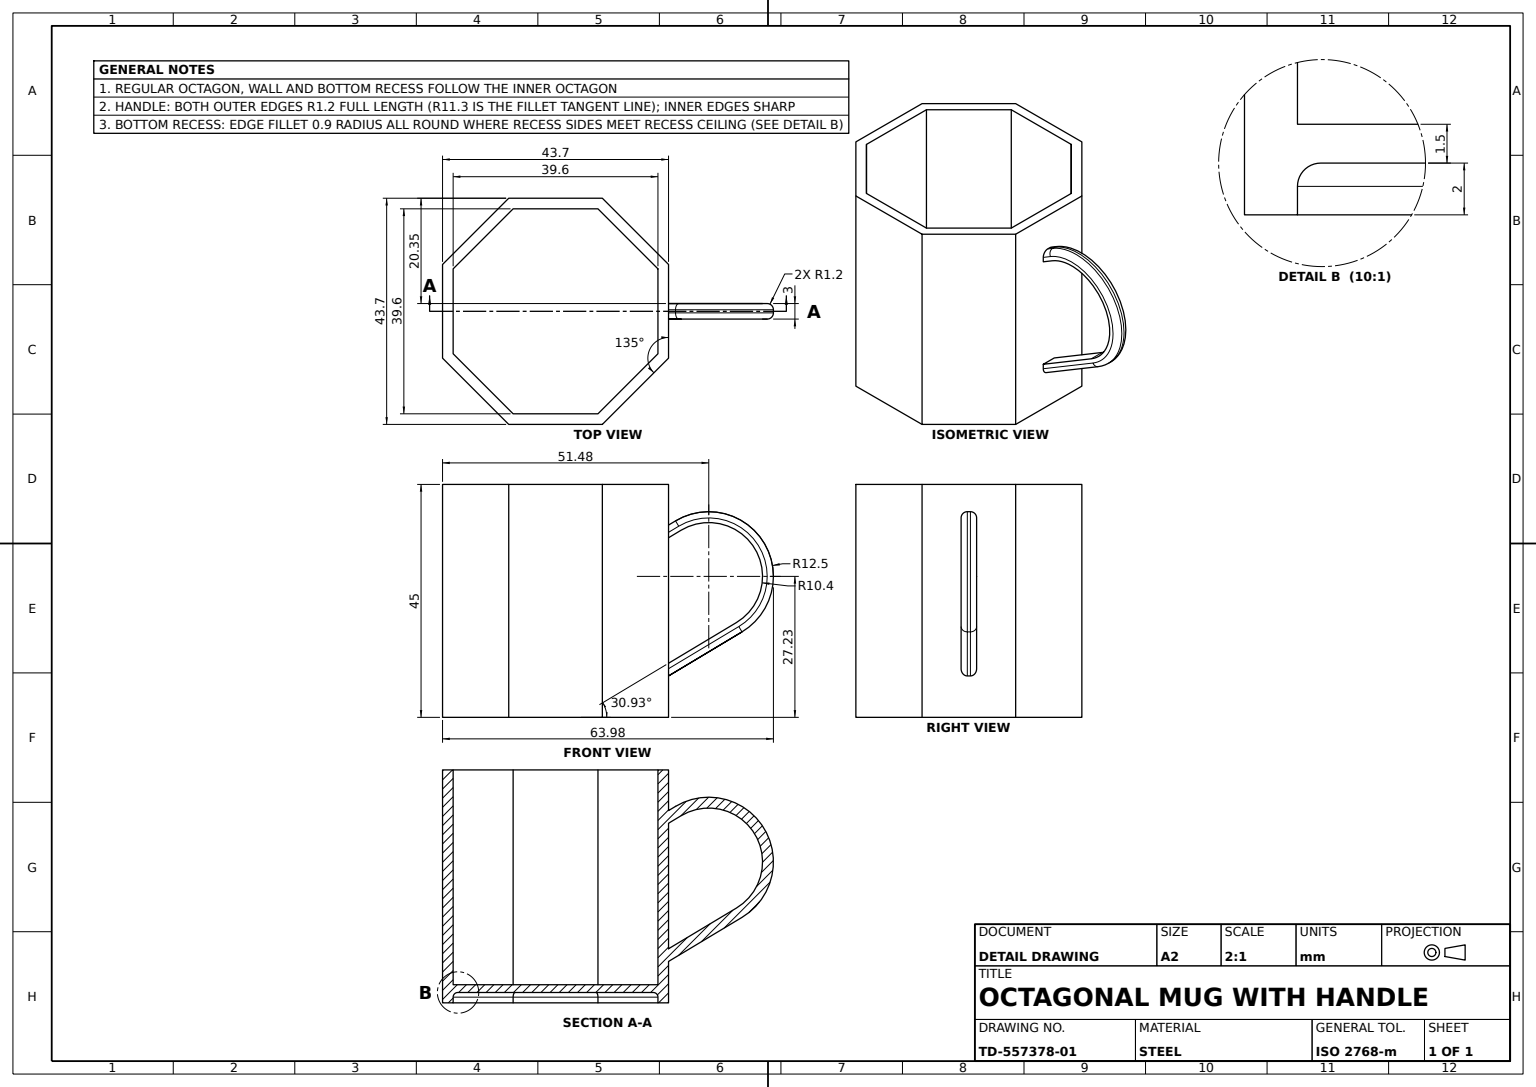
ISO-10303-21;
HEADER;
FILE_DESCRIPTION((''),'2;1');
FILE_NAME('','',(''),(''),'','','');
FILE_SCHEMA(('AUTOMOTIVE_DESIGN'));
ENDSEC;
DATA;
#1=APPLICATION_CONTEXT('');
#2=PRODUCT_CONTEXT('',#1,'mechanical');
#3=PRODUCT('','','',(#2));
#4=PRODUCT_DEFINITION_FORMATION('','',#3);
#5=PRODUCT_DEFINITION_CONTEXT('',#1,'design');
#6=PRODUCT_DEFINITION('','',#4,#5);
#7=PRODUCT_DEFINITION_SHAPE('','',#6);
#8=(LENGTH_UNIT()NAMED_UNIT(*)SI_UNIT(.MILLI.,.METRE.));
#9=(NAMED_UNIT(*)PLANE_ANGLE_UNIT()SI_UNIT($,.RADIAN.));
#10=(NAMED_UNIT(*)SI_UNIT($,.STERADIAN.)SOLID_ANGLE_UNIT());
#11=UNCERTAINTY_MEASURE_WITH_UNIT(LENGTH_MEASURE(1.E-05),#8,'distance_accuracy_value','');
#12=(GEOMETRIC_REPRESENTATION_CONTEXT(3)GLOBAL_UNCERTAINTY_ASSIGNED_CONTEXT((#11))GLOBAL_UNIT_ASSIGNED_CONTEXT((#8,#9,#10))REPRESENTATION_CONTEXT('',''));
#13=CARTESIAN_POINT('',(19.8,-21.4,8.201429));
#14=VERTEX_POINT('',#13);
#15=CARTESIAN_POINT('',(19.8,-22.5,8.201429));
#16=VERTEX_POINT('',#15);
#17=CARTESIAN_POINT('',(19.8,22.5,8.201429));
#18=DIRECTION('',(0.,-1.,0.));
#19=VECTOR('',#18,1000.);
#20=LINE('',#17,#19);
#21=EDGE_CURVE('',#14,#16,#20,.T.);
#22=ORIENTED_EDGE('',*,*,#21,.T.);
#23=CARTESIAN_POINT('',(8.201429,-22.5,19.8));
#24=VERTEX_POINT('',#23);
#25=DIRECTION('',(0.707106781,0.,-0.707106781));
#26=VECTOR('',#25,1000.);
#27=LINE('',#23,#26);
#28=EDGE_CURVE('',#24,#16,#27,.T.);
#29=ORIENTED_EDGE('',*,*,#28,.F.);
#30=CARTESIAN_POINT('',(8.201429,-21.4,19.8));
#31=VERTEX_POINT('',#30);
#32=CARTESIAN_POINT('',(8.201429,22.5,19.8));
#33=LINE('',#32,#19);
#34=EDGE_CURVE('',#31,#24,#33,.T.);
#35=ORIENTED_EDGE('',*,*,#34,.F.);
#36=LINE('',#30,#26);
#37=EDGE_CURVE('',#31,#14,#36,.T.);
#38=ORIENTED_EDGE('',*,*,#37,.T.);
#39=EDGE_LOOP('',(#22,#29,#35,#38));
#40=FACE_OUTER_BOUND('',#39,.T.);
#41=DIRECTION('',(-0.707106781,0.,-0.707106781));
#42=DIRECTION('',(-0.707106781,0.,0.707106781));
#43=AXIS2_PLACEMENT_3D('',#32,#41,#42);
#44=PLANE('',#43);
#45=ADVANCED_FACE('',(#40),#44,.T.);
#46=CARTESIAN_POINT('',(19.8,-21.4,-8.201429));
#47=VERTEX_POINT('',#46);
#48=CARTESIAN_POINT('',(8.201429,-21.4,-19.8));
#49=VERTEX_POINT('',#48);
#50=VECTOR('',#41,1000.);
#51=LINE('',#46,#50);
#52=EDGE_CURVE('',#47,#49,#51,.T.);
#53=ORIENTED_EDGE('',*,*,#52,.F.);
#54=CARTESIAN_POINT('',(18.9,-20.5,-7.828636));
#55=VERTEX_POINT('',#54);
#56=CARTESIAN_POINT('',(19.8,-20.872792,-8.201429));
#57=CARTESIAN_POINT('',(19.427208,-20.5,-8.047013));
#58=(BOUNDED_CURVE()B_SPLINE_CURVE(3,(#46,#56,#57,#54),.UNSPECIFIED.,.F.,.F.)B_SPLINE_CURVE_WITH_KNOTS((4,4),(0.,1.570796327),.UNSPECIFIED.)CURVE()GEOMETRIC_REPRESENTATION_ITEM()RATIONAL_B_SPLINE_CURVE((1.,0.804737854,0.804737854,1.))REPRESENTATION_ITEM(''));
#59=EDGE_CURVE('',#47,#55,#58,.T.);
#60=ORIENTED_EDGE('',*,*,#59,.T.);
#61=CARTESIAN_POINT('',(7.828636,-20.5,-18.9));
#62=VERTEX_POINT('',#61);
#63=CARTESIAN_POINT('',(13.364318,-20.5,-13.364318));
#64=DIRECTION('',(0.707106781,0.,0.707106781));
#65=VECTOR('',#64,1000.);
#66=LINE('',#63,#65);
#67=EDGE_CURVE('',#62,#55,#66,.T.);
#68=ORIENTED_EDGE('',*,*,#67,.F.);
#69=CARTESIAN_POINT('',(8.201429,-20.872792,-19.8));
#70=CARTESIAN_POINT('',(8.047013,-20.5,-19.427208));
#71=(BOUNDED_CURVE()B_SPLINE_CURVE(3,(#48,#69,#70,#61),.UNSPECIFIED.,.F.,.F.)B_SPLINE_CURVE_WITH_KNOTS((4,4),(0.,1.570796327),.UNSPECIFIED.)CURVE()GEOMETRIC_REPRESENTATION_ITEM()RATIONAL_B_SPLINE_CURVE((1.,0.804737854,0.804737854,1.))REPRESENTATION_ITEM(''));
#72=EDGE_CURVE('',#49,#62,#71,.T.);
#73=ORIENTED_EDGE('',*,*,#72,.F.);
#74=EDGE_LOOP('',(#53,#60,#68,#73));
#75=FACE_OUTER_BOUND('',#74,.T.);
#76=CARTESIAN_POINT('',(19.163604,-21.4,-7.565032));
#77=AXIS2_PLACEMENT_3D('',#76,#41,#42);
#78=CYLINDRICAL_SURFACE('',#77,0.9);
#79=ADVANCED_FACE('',(#75),#78,.F.);
#80=CARTESIAN_POINT('',(-8.201429,22.5,19.8));
#81=VERTEX_POINT('',#80);
#82=VERTEX_POINT('',#32);
#83=DIRECTION('',(1.,0.,0.));
#84=VECTOR('',#83,1000.);
#85=LINE('',#80,#84);
#86=EDGE_CURVE('',#81,#82,#85,.T.);
#87=ORIENTED_EDGE('',*,*,#86,.F.);
#88=CARTESIAN_POINT('',(-19.8,22.5,8.201429));
#89=VERTEX_POINT('',#88);
#90=LINE('',#88,#65);
#91=EDGE_CURVE('',#89,#81,#90,.T.);
#92=ORIENTED_EDGE('',*,*,#91,.F.);
#93=CARTESIAN_POINT('',(-19.8,22.5,-8.201429));
#94=VERTEX_POINT('',#93);
#95=DIRECTION('',(0.,0.,1.));
#96=VECTOR('',#95,1000.);
#97=LINE('',#93,#96);
#98=EDGE_CURVE('',#94,#89,#97,.T.);
#99=ORIENTED_EDGE('',*,*,#98,.F.);
#100=CARTESIAN_POINT('',(-8.201429,22.5,-19.8));
#101=VERTEX_POINT('',#100);
#102=VECTOR('',#42,1000.);
#103=LINE('',#100,#102);
#104=EDGE_CURVE('',#101,#94,#103,.T.);
#105=ORIENTED_EDGE('',*,*,#104,.F.);
#106=CARTESIAN_POINT('',(8.201429,22.5,-19.8));
#107=VERTEX_POINT('',#106);
#108=DIRECTION('',(-1.,0.,0.));
#109=VECTOR('',#108,1000.);
#110=LINE('',#106,#109);
#111=EDGE_CURVE('',#107,#101,#110,.T.);
#112=ORIENTED_EDGE('',*,*,#111,.F.);
#113=CARTESIAN_POINT('',(19.8,22.5,-8.201429));
#114=VERTEX_POINT('',#113);
#115=LINE('',#113,#50);
#116=EDGE_CURVE('',#114,#107,#115,.T.);
#117=ORIENTED_EDGE('',*,*,#116,.F.);
#118=VERTEX_POINT('',#17);
#119=DIRECTION('',(0.,0.,-1.));
#120=VECTOR('',#119,1000.);
#121=LINE('',#17,#120);
#122=EDGE_CURVE('',#118,#114,#121,.T.);
#123=ORIENTED_EDGE('',*,*,#122,.F.);
#124=LINE('',#32,#26);
#125=EDGE_CURVE('',#82,#118,#124,.T.);
#126=ORIENTED_EDGE('',*,*,#125,.F.);
#127=EDGE_LOOP('',(#87,#92,#99,#105,#112,#117,#123,#126));
#128=FACE_BOUND('',#127,.T.);
#129=CARTESIAN_POINT('',(9.05,22.5,21.848633));
#130=VERTEX_POINT('',#129);
#131=CARTESIAN_POINT('',(21.848633,22.5,9.05));
#132=VERTEX_POINT('',#131);
#133=LINE('',#129,#26);
#134=EDGE_CURVE('',#130,#132,#133,.T.);
#135=ORIENTED_EDGE('',*,*,#134,.T.);
#136=CARTESIAN_POINT('',(21.848633,22.5,-9.05));
#137=VERTEX_POINT('',#136);
#138=LINE('',#131,#120);
#139=EDGE_CURVE('',#132,#137,#138,.T.);
#140=ORIENTED_EDGE('',*,*,#139,.T.);
#141=CARTESIAN_POINT('',(9.05,22.5,-21.848633));
#142=VERTEX_POINT('',#141);
#143=LINE('',#136,#50);
#144=EDGE_CURVE('',#137,#142,#143,.T.);
#145=ORIENTED_EDGE('',*,*,#144,.T.);
#146=CARTESIAN_POINT('',(-9.05,22.5,-21.848633));
#147=VERTEX_POINT('',#146);
#148=LINE('',#141,#109);
#149=EDGE_CURVE('',#142,#147,#148,.T.);
#150=ORIENTED_EDGE('',*,*,#149,.T.);
#151=CARTESIAN_POINT('',(-21.848633,22.5,-9.05));
#152=VERTEX_POINT('',#151);
#153=LINE('',#146,#102);
#154=EDGE_CURVE('',#147,#152,#153,.T.);
#155=ORIENTED_EDGE('',*,*,#154,.T.);
#156=CARTESIAN_POINT('',(-21.848633,22.5,9.05));
#157=VERTEX_POINT('',#156);
#158=LINE('',#151,#96);
#159=EDGE_CURVE('',#152,#157,#158,.T.);
#160=ORIENTED_EDGE('',*,*,#159,.T.);
#161=CARTESIAN_POINT('',(-9.05,22.5,21.848633));
#162=VERTEX_POINT('',#161);
#163=LINE('',#156,#65);
#164=EDGE_CURVE('',#157,#162,#163,.T.);
#165=ORIENTED_EDGE('',*,*,#164,.T.);
#166=LINE('',#161,#84);
#167=EDGE_CURVE('',#162,#130,#166,.T.);
#168=ORIENTED_EDGE('',*,*,#167,.T.);
#169=EDGE_LOOP('',(#135,#140,#145,#150,#155,#160,#165,#168));
#170=FACE_OUTER_BOUND('',#169,.T.);
#171=CARTESIAN_POINT('',(0.,22.5,0.));
#172=DIRECTION('',(0.,1.,0.));
#173=AXIS2_PLACEMENT_3D('',#171,#172,#95);
#174=PLANE('',#173);
#175=ADVANCED_FACE('',(#128,#170),#174,.T.);
#176=CARTESIAN_POINT('',(-21.848633,-22.5,9.05));
#177=VERTEX_POINT('',#176);
#178=CARTESIAN_POINT('',(-9.05,-22.5,21.848633));
#179=VERTEX_POINT('',#178);
#180=LINE('',#176,#65);
#181=EDGE_CURVE('',#177,#179,#180,.T.);
#182=ORIENTED_EDGE('',*,*,#181,.T.);
#183=LINE('',#161,#19);
#184=EDGE_CURVE('',#162,#179,#183,.T.);
#185=ORIENTED_EDGE('',*,*,#184,.F.);
#186=ORIENTED_EDGE('',*,*,#164,.F.);
#187=LINE('',#156,#19);
#188=EDGE_CURVE('',#157,#177,#187,.T.);
#189=ORIENTED_EDGE('',*,*,#188,.T.);
#190=EDGE_LOOP('',(#182,#185,#186,#189));
#191=FACE_OUTER_BOUND('',#190,.T.);
#192=AXIS2_PLACEMENT_3D('',#156,#25,#41);
#193=PLANE('',#192);
#194=ADVANCED_FACE('',(#191),#193,.F.);
#195=CARTESIAN_POINT('',(36.05233,-5.989286,0.3));
#196=VERTEX_POINT('',#195);
#197=CARTESIAN_POINT('',(36.05233,-5.989286,-0.3));
#198=VERTEX_POINT('',#197);
#199=CARTESIAN_POINT('',(36.05233,-5.989286,1.5));
#200=LINE('',#199,#120);
#201=EDGE_CURVE('',#196,#198,#200,.T.);
#202=ORIENTED_EDGE('',*,*,#201,.F.);
#203=CARTESIAN_POINT('',(21.848633,-14.5,0.3));
#204=VERTEX_POINT('',#203);
#205=DIRECTION('',(-0.857799295,-0.513984796,0.));
#206=VECTOR('',#205,1000.);
#207=LINE('',#203,#206);
#208=EDGE_CURVE('',#196,#204,#207,.T.);
#209=ORIENTED_EDGE('',*,*,#208,.T.);
#210=CARTESIAN_POINT('',(21.848633,-14.5,-0.3));
#211=VERTEX_POINT('',#210);
#212=CARTESIAN_POINT('',(21.848633,-14.5,1.5));
#213=LINE('',#212,#120);
#214=EDGE_CURVE('',#204,#211,#213,.T.);
#215=ORIENTED_EDGE('',*,*,#214,.T.);
#216=DIRECTION('',(0.857799295,0.513984796,0.));
#217=VECTOR('',#216,1000.);
#218=LINE('',#210,#217);
#219=EDGE_CURVE('',#211,#198,#218,.T.);
#220=ORIENTED_EDGE('',*,*,#219,.T.);
#221=EDGE_LOOP('',(#202,#209,#215,#220));
#222=FACE_OUTER_BOUND('',#221,.T.);
#223=DIRECTION('',(-0.513984796,0.857799295,0.));
#224=AXIS2_PLACEMENT_3D('',#212,#223,#205);
#225=PLANE('',#224);
#226=ADVANCED_FACE('',(#222),#225,.F.);
#227=CARTESIAN_POINT('',(8.201429,-22.5,-19.8));
#228=VERTEX_POINT('',#227);
#229=LINE('',#106,#19);
#230=EDGE_CURVE('',#49,#228,#229,.T.);
#231=ORIENTED_EDGE('',*,*,#230,.F.);
#232=CARTESIAN_POINT('',(-8.201429,-21.4,-19.8));
#233=VERTEX_POINT('',#232);
#234=LINE('',#48,#109);
#235=EDGE_CURVE('',#49,#233,#234,.T.);
#236=ORIENTED_EDGE('',*,*,#235,.T.);
#237=CARTESIAN_POINT('',(-8.201429,-22.5,-19.8));
#238=VERTEX_POINT('',#237);
#239=LINE('',#100,#19);
#240=EDGE_CURVE('',#233,#238,#239,.T.);
#241=ORIENTED_EDGE('',*,*,#240,.T.);
#242=LINE('',#227,#109);
#243=EDGE_CURVE('',#228,#238,#242,.T.);
#244=ORIENTED_EDGE('',*,*,#243,.F.);
#245=EDGE_LOOP('',(#231,#236,#241,#244));
#246=FACE_OUTER_BOUND('',#245,.T.);
#247=AXIS2_PLACEMENT_3D('',#106,#95,#83);
#248=PLANE('',#247);
#249=ADVANCED_FACE('',(#246),#248,.T.);
#250=CARTESIAN_POINT('',(-19.8,-21.4,-8.201429));
#251=VERTEX_POINT('',#250);
#252=CARTESIAN_POINT('',(-19.8,-21.4,8.201429));
#253=VERTEX_POINT('',#252);
#254=LINE('',#250,#96);
#255=EDGE_CURVE('',#251,#253,#254,.T.);
#256=ORIENTED_EDGE('',*,*,#255,.T.);
#257=CARTESIAN_POINT('',(-19.8,-22.5,8.201429));
#258=VERTEX_POINT('',#257);
#259=LINE('',#88,#19);
#260=EDGE_CURVE('',#253,#258,#259,.T.);
#261=ORIENTED_EDGE('',*,*,#260,.T.);
#262=CARTESIAN_POINT('',(-19.8,-22.5,-8.201429));
#263=VERTEX_POINT('',#262);
#264=LINE('',#262,#96);
#265=EDGE_CURVE('',#263,#258,#264,.T.);
#266=ORIENTED_EDGE('',*,*,#265,.F.);
#267=LINE('',#93,#19);
#268=EDGE_CURVE('',#251,#263,#267,.T.);
#269=ORIENTED_EDGE('',*,*,#268,.F.);
#270=EDGE_LOOP('',(#256,#261,#266,#269));
#271=FACE_OUTER_BOUND('',#270,.T.);
#272=AXIS2_PLACEMENT_3D('',#93,#83,#119);
#273=PLANE('',#272);
#274=ADVANCED_FACE('',(#271),#273,.T.);
#275=CARTESIAN_POINT('',(-19.8,-19.,-8.201429));
#276=VERTEX_POINT('',#275);
#277=EDGE_CURVE('',#94,#276,#267,.T.);
#278=ORIENTED_EDGE('',*,*,#277,.T.);
#279=CARTESIAN_POINT('',(-8.201429,-19.,-19.8));
#280=VERTEX_POINT('',#279);
#281=LINE('',#279,#102);
#282=EDGE_CURVE('',#280,#276,#281,.T.);
#283=ORIENTED_EDGE('',*,*,#282,.F.);
#284=EDGE_CURVE('',#101,#280,#239,.T.);
#285=ORIENTED_EDGE('',*,*,#284,.F.);
#286=ORIENTED_EDGE('',*,*,#104,.T.);
#287=EDGE_LOOP('',(#278,#283,#285,#286));
#288=FACE_OUTER_BOUND('',#287,.T.);
#289=AXIS2_PLACEMENT_3D('',#100,#64,#25);
#290=PLANE('',#289);
#291=ADVANCED_FACE('',(#288),#290,.T.);
#292=CARTESIAN_POINT('',(-18.9,-20.5,-7.828636));
#293=VERTEX_POINT('',#292);
#294=CARTESIAN_POINT('',(-7.828636,-20.5,-18.9));
#295=VERTEX_POINT('',#294);
#296=CARTESIAN_POINT('',(-13.364318,-20.5,-13.364318));
#297=LINE('',#296,#26);
#298=EDGE_CURVE('',#293,#295,#297,.T.);
#299=ORIENTED_EDGE('',*,*,#298,.F.);
#300=CARTESIAN_POINT('',(-19.8,-20.872792,-8.201429));
#301=CARTESIAN_POINT('',(-19.427208,-20.5,-8.047013));
#302=(BOUNDED_CURVE()B_SPLINE_CURVE(3,(#250,#300,#301,#292),.UNSPECIFIED.,.F.,.F.)B_SPLINE_CURVE_WITH_KNOTS((4,4),(3.141592654,4.71238898),.UNSPECIFIED.)CURVE()GEOMETRIC_REPRESENTATION_ITEM()RATIONAL_B_SPLINE_CURVE((1.,0.804737854,0.804737854,1.))REPRESENTATION_ITEM(''));
#303=EDGE_CURVE('',#251,#293,#302,.T.);
#304=ORIENTED_EDGE('',*,*,#303,.F.);
#305=LINE('',#232,#102);
#306=EDGE_CURVE('',#233,#251,#305,.T.);
#307=ORIENTED_EDGE('',*,*,#306,.F.);
#308=CARTESIAN_POINT('',(-8.201429,-20.872792,-19.8));
#309=CARTESIAN_POINT('',(-8.047013,-20.5,-19.427208));
#310=(BOUNDED_CURVE()B_SPLINE_CURVE(3,(#232,#308,#309,#294),.UNSPECIFIED.,.F.,.F.)B_SPLINE_CURVE_WITH_KNOTS((4,4),(0.,1.570796327),.UNSPECIFIED.)CURVE()GEOMETRIC_REPRESENTATION_ITEM()RATIONAL_B_SPLINE_CURVE((1.,0.804737854,0.804737854,1.))REPRESENTATION_ITEM(''));
#311=EDGE_CURVE('',#233,#295,#310,.T.);
#312=ORIENTED_EDGE('',*,*,#311,.T.);
#313=EDGE_LOOP('',(#299,#304,#307,#312));
#314=FACE_OUTER_BOUND('',#313,.T.);
#315=CARTESIAN_POINT('',(-7.565032,-21.4,-19.163604));
#316=AXIS2_PLACEMENT_3D('',#315,#42,#64);
#317=CYLINDRICAL_SURFACE('',#316,0.9);
#318=ADVANCED_FACE('',(#314),#317,.F.);
#319=CARTESIAN_POINT('',(42.12752,4.733205,-0.3));
#320=VERTEX_POINT('',#319);
#321=CARTESIAN_POINT('',(29.62752,4.733205,-0.3));
#322=AXIS2_PLACEMENT_3D('',#321,#95,#83);
#323=CIRCLE('',#322,12.5);
#324=EDGE_CURVE('',#198,#320,#323,.T.);
#325=ORIENTED_EDGE('',*,*,#324,.F.);
#326=CARTESIAN_POINT('',(35.435548,-4.959927,-1.5));
#327=VERTEX_POINT('',#326);
#328=CARTESIAN_POINT('',(35.435548,-4.959927,-0.3));
#329=DIRECTION('',(0.513984796,-0.857799295,0.));
#330=AXIS2_PLACEMENT_3D('',#328,#205,#329);
#331=CIRCLE('',#330,1.2);
#332=EDGE_CURVE('',#327,#198,#331,.T.);
#333=ORIENTED_EDGE('',*,*,#332,.F.);
#334=CARTESIAN_POINT('',(40.92752,4.733205,-1.5));
#335=VERTEX_POINT('',#334);
#336=CARTESIAN_POINT('',(29.62752,4.733205,-1.5));
#337=AXIS2_PLACEMENT_3D('',#336,#119,#83);
#338=CIRCLE('',#337,11.3);
#339=EDGE_CURVE('',#335,#327,#338,.T.);
#340=ORIENTED_EDGE('',*,*,#339,.F.);
#341=CARTESIAN_POINT('',(40.92752,4.733205,-0.3));
#342=AXIS2_PLACEMENT_3D('',#341,#18,#119);
#343=CIRCLE('',#342,1.2);
#344=EDGE_CURVE('',#335,#320,#343,.T.);
#345=ORIENTED_EDGE('',*,*,#344,.T.);
#346=EDGE_LOOP('',(#325,#333,#340,#345));
#347=FACE_OUTER_BOUND('',#346,.T.);
#348=TOROIDAL_SURFACE('',#322,11.3,1.2);
#349=ADVANCED_FACE('',(#347),#348,.T.);
#350=ORIENTED_EDGE('',*,*,#260,.F.);
#351=CARTESIAN_POINT('',(-8.201429,-21.4,19.8));
#352=VERTEX_POINT('',#351);
#353=LINE('',#252,#65);
#354=EDGE_CURVE('',#253,#352,#353,.T.);
#355=ORIENTED_EDGE('',*,*,#354,.T.);
#356=CARTESIAN_POINT('',(-8.201429,-22.5,19.8));
#357=VERTEX_POINT('',#356);
#358=LINE('',#80,#19);
#359=EDGE_CURVE('',#352,#357,#358,.T.);
#360=ORIENTED_EDGE('',*,*,#359,.T.);
#361=LINE('',#257,#65);
#362=EDGE_CURVE('',#258,#357,#361,.T.);
#363=ORIENTED_EDGE('',*,*,#362,.F.);
#364=EDGE_LOOP('',(#350,#355,#360,#363));
#365=FACE_OUTER_BOUND('',#364,.T.);
#366=AXIS2_PLACEMENT_3D('',#88,#25,#41);
#367=PLANE('',#366);
#368=ADVANCED_FACE('',(#365),#367,.T.);
#369=CARTESIAN_POINT('',(21.848633,13.245418,1.5));
#370=VERTEX_POINT('',#369);
#371=CARTESIAN_POINT('',(21.848633,14.644347,0.3));
#372=VERTEX_POINT('',#371);
#373=CARTESIAN_POINT('',(21.848633,14.064891,1.5));
#374=CARTESIAN_POINT('',(21.848633,14.644347,1.002944));
#375=(BOUNDED_CURVE()B_SPLINE_CURVE(3,(#369,#373,#374,#371),.UNSPECIFIED.,.F.,.F.)B_SPLINE_CURVE_WITH_KNOTS((4,4),(4.71238898,6.283185307),.UNSPECIFIED.)CURVE()GEOMETRIC_REPRESENTATION_ITEM()RATIONAL_B_SPLINE_CURVE((1.,0.804737854,0.804737854,1.))REPRESENTATION_ITEM(''));
#376=EDGE_CURVE('',#370,#372,#375,.T.);
#377=ORIENTED_EDGE('',*,*,#376,.T.);
#378=CARTESIAN_POINT('',(21.848633,14.644347,-0.3));
#379=VERTEX_POINT('',#378);
#380=CARTESIAN_POINT('',(21.848633,14.644347,1.5));
#381=LINE('',#380,#120);
#382=EDGE_CURVE('',#372,#379,#381,.T.);
#383=ORIENTED_EDGE('',*,*,#382,.T.);
#384=CARTESIAN_POINT('',(21.848633,13.245418,-1.5));
#385=VERTEX_POINT('',#384);
#386=CARTESIAN_POINT('',(21.848633,14.644347,-1.002944));
#387=CARTESIAN_POINT('',(21.848633,14.064891,-1.5));
#388=(BOUNDED_CURVE()B_SPLINE_CURVE(3,(#378,#386,#387,#384),.UNSPECIFIED.,.F.,.T.)B_SPLINE_CURVE_WITH_KNOTS((4,4),(3.141592654,4.71238898),.UNSPECIFIED.)CURVE()GEOMETRIC_REPRESENTATION_ITEM()RATIONAL_B_SPLINE_CURVE((1.,0.804737854,0.804737854,1.))REPRESENTATION_ITEM(''));
#389=EDGE_CURVE('',#379,#385,#388,.T.);
#390=ORIENTED_EDGE('',*,*,#389,.T.);
#391=CARTESIAN_POINT('',(21.848633,12.196222,-1.5));
#392=VERTEX_POINT('',#391);
#393=LINE('',#391,#19);
#394=EDGE_CURVE('',#385,#392,#393,.T.);
#395=ORIENTED_EDGE('',*,*,#394,.T.);
#396=CARTESIAN_POINT('',(21.848633,12.196222,1.5));
#397=VERTEX_POINT('',#396);
#398=LINE('',#396,#120);
#399=EDGE_CURVE('',#397,#392,#398,.T.);
#400=ORIENTED_EDGE('',*,*,#399,.F.);
#401=LINE('',#396,#19);
#402=EDGE_CURVE('',#370,#397,#401,.T.);
#403=ORIENTED_EDGE('',*,*,#402,.F.);
#404=EDGE_LOOP('',(#377,#383,#390,#395,#400,#403));
#405=FACE_BOUND('',#404,.T.);
#406=CARTESIAN_POINT('',(21.848633,-22.5,9.05));
#407=VERTEX_POINT('',#406);
#408=CARTESIAN_POINT('',(21.848633,-22.5,-9.05));
#409=VERTEX_POINT('',#408);
#410=LINE('',#406,#120);
#411=EDGE_CURVE('',#407,#409,#410,.T.);
#412=ORIENTED_EDGE('',*,*,#411,.T.);
#413=LINE('',#136,#19);
#414=EDGE_CURVE('',#137,#409,#413,.T.);
#415=ORIENTED_EDGE('',*,*,#414,.F.);
#416=ORIENTED_EDGE('',*,*,#139,.F.);
#417=LINE('',#131,#19);
#418=EDGE_CURVE('',#132,#407,#417,.T.);
#419=ORIENTED_EDGE('',*,*,#418,.T.);
#420=EDGE_LOOP('',(#412,#415,#416,#419));
#421=FACE_OUTER_BOUND('',#420,.T.);
#422=CARTESIAN_POINT('',(21.848633,-13.101071,-1.5));
#423=VERTEX_POINT('',#422);
#424=CARTESIAN_POINT('',(21.848633,-13.920545,-1.5));
#425=CARTESIAN_POINT('',(21.848633,-14.5,-1.002944));
#426=(BOUNDED_CURVE()B_SPLINE_CURVE(3,(#422,#424,#425,#210),.UNSPECIFIED.,.F.,.F.)B_SPLINE_CURVE_WITH_KNOTS((4,4),(1.570796327,3.141592654),.UNSPECIFIED.)CURVE()GEOMETRIC_REPRESENTATION_ITEM()RATIONAL_B_SPLINE_CURVE((1.,0.804737854,0.804737854,1.))REPRESENTATION_ITEM(''));
#427=EDGE_CURVE('',#423,#211,#426,.T.);
#428=ORIENTED_EDGE('',*,*,#427,.T.);
#429=ORIENTED_EDGE('',*,*,#214,.F.);
#430=CARTESIAN_POINT('',(21.848633,-13.101071,1.5));
#431=VERTEX_POINT('',#430);
#432=CARTESIAN_POINT('',(21.848633,-14.5,1.002944));
#433=CARTESIAN_POINT('',(21.848633,-13.920545,1.5));
#434=(BOUNDED_CURVE()B_SPLINE_CURVE(3,(#203,#432,#433,#430),.UNSPECIFIED.,.F.,.F.)B_SPLINE_CURVE_WITH_KNOTS((4,4),(0.,1.570796327),.UNSPECIFIED.)CURVE()GEOMETRIC_REPRESENTATION_ITEM()RATIONAL_B_SPLINE_CURVE((1.,0.804737854,0.804737854,1.))REPRESENTATION_ITEM(''));
#435=EDGE_CURVE('',#204,#431,#434,.T.);
#436=ORIENTED_EDGE('',*,*,#435,.T.);
#437=CARTESIAN_POINT('',(21.848633,-12.051875,1.5));
#438=VERTEX_POINT('',#437);
#439=LINE('',#212,#19);
#440=EDGE_CURVE('',#438,#431,#439,.T.);
#441=ORIENTED_EDGE('',*,*,#440,.F.);
#442=CARTESIAN_POINT('',(21.848633,-12.051875,-1.5));
#443=VERTEX_POINT('',#442);
#444=LINE('',#437,#120);
#445=EDGE_CURVE('',#438,#443,#444,.T.);
#446=ORIENTED_EDGE('',*,*,#445,.T.);
#447=CARTESIAN_POINT('',(21.848633,-14.5,-1.5));
#448=LINE('',#447,#19);
#449=EDGE_CURVE('',#443,#423,#448,.T.);
#450=ORIENTED_EDGE('',*,*,#449,.T.);
#451=EDGE_LOOP('',(#428,#429,#436,#441,#446,#450));
#452=FACE_BOUND('',#451,.T.);
#453=AXIS2_PLACEMENT_3D('',#131,#108,#95);
#454=PLANE('',#453);
#455=ADVANCED_FACE('',(#405,#421,#452),#454,.F.);
#456=ORIENTED_EDGE('',*,*,#303,.T.);
#457=CARTESIAN_POINT('',(-18.9,-20.5,7.828636));
#458=VERTEX_POINT('',#457);
#459=CARTESIAN_POINT('',(-18.9,-20.5,0.));
#460=LINE('',#459,#120);
#461=EDGE_CURVE('',#458,#293,#460,.T.);
#462=ORIENTED_EDGE('',*,*,#461,.F.);
#463=CARTESIAN_POINT('',(-19.427208,-20.5,8.047013));
#464=CARTESIAN_POINT('',(-19.8,-20.872792,8.201429));
#465=(BOUNDED_CURVE()B_SPLINE_CURVE(3,(#457,#463,#464,#252),.UNSPECIFIED.,.F.,.F.)B_SPLINE_CURVE_WITH_KNOTS((4,4),(4.71238898,6.283185307),.UNSPECIFIED.)CURVE()GEOMETRIC_REPRESENTATION_ITEM()RATIONAL_B_SPLINE_CURVE((1.,0.804737854,0.804737854,1.))REPRESENTATION_ITEM(''));
#466=EDGE_CURVE('',#458,#253,#465,.T.);
#467=ORIENTED_EDGE('',*,*,#466,.T.);
#468=ORIENTED_EDGE('',*,*,#255,.F.);
#469=EDGE_LOOP('',(#456,#462,#467,#468));
#470=FACE_OUTER_BOUND('',#469,.T.);
#471=CARTESIAN_POINT('',(-18.9,-21.4,-8.201429));
#472=AXIS2_PLACEMENT_3D('',#471,#95,#83);
#473=CYLINDRICAL_SURFACE('',#472,0.9);
#474=ADVANCED_FACE('',(#470),#473,.F.);
#475=CARTESIAN_POINT('',(8.201429,-19.,19.8));
#476=VERTEX_POINT('',#475);
#477=CARTESIAN_POINT('',(19.8,-19.,8.201429));
#478=VERTEX_POINT('',#477);
#479=LINE('',#475,#26);
#480=EDGE_CURVE('',#476,#478,#479,.T.);
#481=ORIENTED_EDGE('',*,*,#480,.F.);
#482=EDGE_CURVE('',#82,#476,#33,.T.);
#483=ORIENTED_EDGE('',*,*,#482,.F.);
#484=ORIENTED_EDGE('',*,*,#125,.T.);
#485=EDGE_CURVE('',#118,#478,#20,.T.);
#486=ORIENTED_EDGE('',*,*,#485,.T.);
#487=EDGE_LOOP('',(#481,#483,#484,#486));
#488=FACE_OUTER_BOUND('',#487,.T.);
#489=ADVANCED_FACE('',(#488),#44,.T.);
#490=CARTESIAN_POINT('',(19.8,-19.,-8.201429));
#491=VERTEX_POINT('',#490);
#492=LINE('',#113,#19);
#493=EDGE_CURVE('',#114,#491,#492,.T.);
#494=ORIENTED_EDGE('',*,*,#493,.T.);
#495=LINE('',#477,#120);
#496=EDGE_CURVE('',#478,#491,#495,.T.);
#497=ORIENTED_EDGE('',*,*,#496,.F.);
#498=ORIENTED_EDGE('',*,*,#485,.F.);
#499=ORIENTED_EDGE('',*,*,#122,.T.);
#500=EDGE_LOOP('',(#494,#497,#498,#499));
#501=FACE_OUTER_BOUND('',#500,.T.);
#502=AXIS2_PLACEMENT_3D('',#17,#108,#95);
#503=PLANE('',#502);
#504=ADVANCED_FACE('',(#501),#503,.T.);
#505=CARTESIAN_POINT('',(24.282078,13.654318,-1.5));
#506=VERTEX_POINT('',#505);
#507=CARTESIAN_POINT('',(34.972962,-4.187908,-1.5));
#508=VERTEX_POINT('',#507);
#509=CIRCLE('',#337,10.4);
#510=EDGE_CURVE('',#506,#508,#509,.T.);
#511=ORIENTED_EDGE('',*,*,#510,.T.);
#512=CARTESIAN_POINT('',(34.972962,-4.187908,1.5));
#513=VERTEX_POINT('',#512);
#514=LINE('',#512,#120);
#515=EDGE_CURVE('',#513,#508,#514,.T.);
#516=ORIENTED_EDGE('',*,*,#515,.F.);
#517=CARTESIAN_POINT('',(24.282078,13.654318,1.5));
#518=VERTEX_POINT('',#517);
#519=CARTESIAN_POINT('',(29.62752,4.733205,1.5));
#520=AXIS2_PLACEMENT_3D('',#519,#119,#83);
#521=CIRCLE('',#520,10.4);
#522=EDGE_CURVE('',#518,#513,#521,.T.);
#523=ORIENTED_EDGE('',*,*,#522,.F.);
#524=LINE('',#517,#120);
#525=EDGE_CURVE('',#518,#506,#524,.T.);
#526=ORIENTED_EDGE('',*,*,#525,.T.);
#527=EDGE_LOOP('',(#511,#516,#523,#526));
#528=FACE_OUTER_BOUND('',#527,.T.);
#529=AXIS2_PLACEMENT_3D('',#519,#119,#108);
#530=CYLINDRICAL_SURFACE('',#529,10.4);
#531=ADVANCED_FACE('',(#528),#530,.F.);
#532=ORIENTED_EDGE('',*,*,#21,.F.);
#533=LINE('',#13,#120);
#534=EDGE_CURVE('',#14,#47,#533,.T.);
#535=ORIENTED_EDGE('',*,*,#534,.T.);
#536=CARTESIAN_POINT('',(19.8,-22.5,-8.201429));
#537=VERTEX_POINT('',#536);
#538=EDGE_CURVE('',#47,#537,#492,.T.);
#539=ORIENTED_EDGE('',*,*,#538,.T.);
#540=LINE('',#15,#120);
#541=EDGE_CURVE('',#16,#537,#540,.T.);
#542=ORIENTED_EDGE('',*,*,#541,.F.);
#543=EDGE_LOOP('',(#532,#535,#539,#542));
#544=FACE_OUTER_BOUND('',#543,.T.);
#545=ADVANCED_FACE('',(#544),#503,.T.);
#546=LINE('',#536,#50);
#547=EDGE_CURVE('',#537,#228,#546,.T.);
#548=ORIENTED_EDGE('',*,*,#547,.F.);
#549=ORIENTED_EDGE('',*,*,#538,.F.);
#550=ORIENTED_EDGE('',*,*,#52,.T.);
#551=ORIENTED_EDGE('',*,*,#230,.T.);
#552=EDGE_LOOP('',(#548,#549,#550,#551));
#553=FACE_OUTER_BOUND('',#552,.T.);
#554=AXIS2_PLACEMENT_3D('',#113,#42,#64);
#555=PLANE('',#554);
#556=ADVANCED_FACE('',(#553),#555,.T.);
#557=ORIENTED_EDGE('',*,*,#435,.F.);
#558=ORIENTED_EDGE('',*,*,#208,.F.);
#559=CARTESIAN_POINT('',(35.435548,-4.959927,1.5));
#560=VERTEX_POINT('',#559);
#561=CARTESIAN_POINT('',(35.435548,-4.959927,0.3));
#562=AXIS2_PLACEMENT_3D('',#561,#205,#329);
#563=CIRCLE('',#562,1.2);
#564=EDGE_CURVE('',#196,#560,#563,.T.);
#565=ORIENTED_EDGE('',*,*,#564,.T.);
#566=LINE('',#559,#217);
#567=EDGE_CURVE('',#431,#560,#566,.T.);
#568=ORIENTED_EDGE('',*,*,#567,.F.);
#569=EDGE_LOOP('',(#557,#558,#565,#568));
#570=FACE_OUTER_BOUND('',#569,.T.);
#571=CYLINDRICAL_SURFACE('',#562,1.2);
#572=ADVANCED_FACE('',(#570),#571,.T.);
#573=CARTESIAN_POINT('',(-8.201429,-19.,19.8));
#574=VERTEX_POINT('',#573);
#575=LINE('',#573,#84);
#576=EDGE_CURVE('',#574,#476,#575,.T.);
#577=ORIENTED_EDGE('',*,*,#576,.F.);
#578=EDGE_CURVE('',#81,#574,#358,.T.);
#579=ORIENTED_EDGE('',*,*,#578,.F.);
#580=ORIENTED_EDGE('',*,*,#86,.T.);
#581=ORIENTED_EDGE('',*,*,#482,.T.);
#582=EDGE_LOOP('',(#577,#579,#580,#581));
#583=FACE_OUTER_BOUND('',#582,.T.);
#584=AXIS2_PLACEMENT_3D('',#80,#119,#108);
#585=PLANE('',#584);
#586=ADVANCED_FACE('',(#583),#585,.T.);
#587=ORIENTED_EDGE('',*,*,#159,.F.);
#588=CARTESIAN_POINT('',(-21.848633,-22.5,-9.05));
#589=VERTEX_POINT('',#588);
#590=LINE('',#151,#19);
#591=EDGE_CURVE('',#152,#589,#590,.T.);
#592=ORIENTED_EDGE('',*,*,#591,.T.);
#593=LINE('',#588,#96);
#594=EDGE_CURVE('',#589,#177,#593,.T.);
#595=ORIENTED_EDGE('',*,*,#594,.T.);
#596=ORIENTED_EDGE('',*,*,#188,.F.);
#597=EDGE_LOOP('',(#587,#592,#595,#596));
#598=FACE_OUTER_BOUND('',#597,.T.);
#599=AXIS2_PLACEMENT_3D('',#151,#83,#119);
#600=PLANE('',#599);
#601=ADVANCED_FACE('',(#598),#600,.F.);
#602=CARTESIAN_POINT('',(23.20271,15.455696,-0.3));
#603=VERTEX_POINT('',#602);
#604=LINE('',#602,#206);
#605=EDGE_CURVE('',#603,#379,#604,.T.);
#606=ORIENTED_EDGE('',*,*,#605,.F.);
#607=CARTESIAN_POINT('',(23.819492,14.426337,-1.5));
#608=VERTEX_POINT('',#607);
#609=CARTESIAN_POINT('',(23.819492,14.426337,-0.3));
#610=AXIS2_PLACEMENT_3D('',#609,#216,#223);
#611=CIRCLE('',#610,1.2);
#612=EDGE_CURVE('',#608,#603,#611,.T.);
#613=ORIENTED_EDGE('',*,*,#612,.F.);
#614=LINE('',#607,#217);
#615=EDGE_CURVE('',#385,#608,#614,.T.);
#616=ORIENTED_EDGE('',*,*,#615,.F.);
#617=ORIENTED_EDGE('',*,*,#389,.F.);
#618=EDGE_LOOP('',(#606,#613,#616,#617));
#619=FACE_OUTER_BOUND('',#618,.T.);
#620=AXIS2_PLACEMENT_3D('',#609,#205,#329);
#621=CYLINDRICAL_SURFACE('',#620,1.2);
#622=ADVANCED_FACE('',(#619),#621,.T.);
#623=ORIENTED_EDGE('',*,*,#515,.T.);
#624=LINE('',#442,#206);
#625=EDGE_CURVE('',#508,#443,#624,.T.);
#626=ORIENTED_EDGE('',*,*,#625,.T.);
#627=ORIENTED_EDGE('',*,*,#445,.F.);
#628=LINE('',#437,#206);
#629=EDGE_CURVE('',#513,#438,#628,.T.);
#630=ORIENTED_EDGE('',*,*,#629,.F.);
#631=EDGE_LOOP('',(#623,#626,#627,#630));
#632=FACE_OUTER_BOUND('',#631,.T.);
#633=AXIS2_PLACEMENT_3D('',#437,#329,#216);
#634=PLANE('',#633);
#635=ADVANCED_FACE('',(#632),#634,.F.);
#636=CARTESIAN_POINT('',(42.12752,4.733205,0.3));
#637=VERTEX_POINT('',#636);
#638=CARTESIAN_POINT('',(29.62752,4.733205,0.3));
#639=AXIS2_PLACEMENT_3D('',#638,#119,#83);
#640=CIRCLE('',#639,12.5);
#641=EDGE_CURVE('',#637,#196,#640,.T.);
#642=ORIENTED_EDGE('',*,*,#641,.F.);
#643=CARTESIAN_POINT('',(40.92752,4.733205,1.5));
#644=VERTEX_POINT('',#643);
#645=CARTESIAN_POINT('',(40.92752,4.733205,0.3));
#646=AXIS2_PLACEMENT_3D('',#645,#18,#119);
#647=CIRCLE('',#646,1.2);
#648=EDGE_CURVE('',#637,#644,#647,.T.);
#649=ORIENTED_EDGE('',*,*,#648,.T.);
#650=AXIS2_PLACEMENT_3D('',#519,#95,#83);
#651=CIRCLE('',#650,11.3);
#652=EDGE_CURVE('',#560,#644,#651,.T.);
#653=ORIENTED_EDGE('',*,*,#652,.F.);
#654=ORIENTED_EDGE('',*,*,#564,.F.);
#655=EDGE_LOOP('',(#642,#649,#653,#654));
#656=FACE_OUTER_BOUND('',#655,.T.);
#657=AXIS2_PLACEMENT_3D('',#638,#95,#83);
#658=TOROIDAL_SURFACE('',#657,11.3,1.2);
#659=ADVANCED_FACE('',(#656),#658,.T.);
#660=CARTESIAN_POINT('',(-19.8,-19.,8.201429));
#661=VERTEX_POINT('',#660);
#662=LINE('',#660,#65);
#663=EDGE_CURVE('',#661,#574,#662,.T.);
#664=ORIENTED_EDGE('',*,*,#663,.T.);
#665=ORIENTED_EDGE('',*,*,#576,.T.);
#666=ORIENTED_EDGE('',*,*,#480,.T.);
#667=ORIENTED_EDGE('',*,*,#496,.T.);
#668=CARTESIAN_POINT('',(8.201429,-19.,-19.8));
#669=VERTEX_POINT('',#668);
#670=LINE('',#490,#50);
#671=EDGE_CURVE('',#491,#669,#670,.T.);
#672=ORIENTED_EDGE('',*,*,#671,.T.);
#673=LINE('',#668,#109);
#674=EDGE_CURVE('',#669,#280,#673,.T.);
#675=ORIENTED_EDGE('',*,*,#674,.T.);
#676=ORIENTED_EDGE('',*,*,#282,.T.);
#677=LINE('',#275,#96);
#678=EDGE_CURVE('',#276,#661,#677,.T.);
#679=ORIENTED_EDGE('',*,*,#678,.T.);
#680=EDGE_LOOP('',(#664,#665,#666,#667,#672,#675,#676,#679));
#681=FACE_OUTER_BOUND('',#680,.T.);
#682=CARTESIAN_POINT('',(0.,-19.,0.));
#683=AXIS2_PLACEMENT_3D('',#682,#172,#95);
#684=PLANE('',#683);
#685=ADVANCED_FACE('',(#681),#684,.T.);
#686=ORIENTED_EDGE('',*,*,#376,.F.);
#687=CARTESIAN_POINT('',(23.819492,14.426337,1.5));
#688=VERTEX_POINT('',#687);
#689=CARTESIAN_POINT('',(22.465414,13.614987,1.5));
#690=LINE('',#689,#206);
#691=EDGE_CURVE('',#688,#370,#690,.T.);
#692=ORIENTED_EDGE('',*,*,#691,.F.);
#693=CARTESIAN_POINT('',(23.20271,15.455696,0.3));
#694=VERTEX_POINT('',#693);
#695=CARTESIAN_POINT('',(23.819492,14.426337,0.3));
#696=AXIS2_PLACEMENT_3D('',#695,#216,#223);
#697=CIRCLE('',#696,1.2);
#698=EDGE_CURVE('',#694,#688,#697,.T.);
#699=ORIENTED_EDGE('',*,*,#698,.F.);
#700=LINE('',#693,#217);
#701=EDGE_CURVE('',#372,#694,#700,.T.);
#702=ORIENTED_EDGE('',*,*,#701,.F.);
#703=EDGE_LOOP('',(#686,#692,#699,#702));
#704=FACE_OUTER_BOUND('',#703,.T.);
#705=CYLINDRICAL_SURFACE('',#696,1.2);
#706=ADVANCED_FACE('',(#704),#705,.T.);
#707=ORIENTED_EDGE('',*,*,#184,.T.);
#708=CARTESIAN_POINT('',(9.05,-22.5,21.848633));
#709=VERTEX_POINT('',#708);
#710=LINE('',#178,#84);
#711=EDGE_CURVE('',#179,#709,#710,.T.);
#712=ORIENTED_EDGE('',*,*,#711,.T.);
#713=LINE('',#129,#19);
#714=EDGE_CURVE('',#130,#709,#713,.T.);
#715=ORIENTED_EDGE('',*,*,#714,.F.);
#716=ORIENTED_EDGE('',*,*,#167,.F.);
#717=EDGE_LOOP('',(#707,#712,#715,#716));
#718=FACE_OUTER_BOUND('',#717,.T.);
#719=AXIS2_PLACEMENT_3D('',#161,#119,#108);
#720=PLANE('',#719);
#721=ADVANCED_FACE('',(#718),#720,.F.);
#722=ORIENTED_EDGE('',*,*,#652,.T.);
#723=EDGE_CURVE('',#644,#688,#651,.T.);
#724=ORIENTED_EDGE('',*,*,#723,.T.);
#725=ORIENTED_EDGE('',*,*,#691,.T.);
#726=ORIENTED_EDGE('',*,*,#402,.T.);
#727=LINE('',#517,#217);
#728=EDGE_CURVE('',#397,#518,#727,.T.);
#729=ORIENTED_EDGE('',*,*,#728,.T.);
#730=ORIENTED_EDGE('',*,*,#522,.T.);
#731=ORIENTED_EDGE('',*,*,#629,.T.);
#732=ORIENTED_EDGE('',*,*,#440,.T.);
#733=ORIENTED_EDGE('',*,*,#567,.T.);
#734=EDGE_LOOP('',(#722,#724,#725,#726,#729,#730,#731,#732,#733));
#735=FACE_OUTER_BOUND('',#734,.T.);
#736=PLANE('',#650);
#737=ADVANCED_FACE('',(#735),#736,.T.);
#738=ORIENTED_EDGE('',*,*,#354,.F.);
#739=ORIENTED_EDGE('',*,*,#466,.F.);
#740=CARTESIAN_POINT('',(-7.828636,-20.5,18.9));
#741=VERTEX_POINT('',#740);
#742=CARTESIAN_POINT('',(-13.364318,-20.5,13.364318));
#743=LINE('',#742,#50);
#744=EDGE_CURVE('',#741,#458,#743,.T.);
#745=ORIENTED_EDGE('',*,*,#744,.F.);
#746=CARTESIAN_POINT('',(-8.047013,-20.5,19.427208));
#747=CARTESIAN_POINT('',(-8.201429,-20.872792,19.8));
#748=(BOUNDED_CURVE()B_SPLINE_CURVE(3,(#740,#746,#747,#351),.UNSPECIFIED.,.F.,.F.)B_SPLINE_CURVE_WITH_KNOTS((4,4),(4.71238898,6.283185307),.UNSPECIFIED.)CURVE()GEOMETRIC_REPRESENTATION_ITEM()RATIONAL_B_SPLINE_CURVE((1.,0.804737854,0.804737854,1.))REPRESENTATION_ITEM(''));
#749=EDGE_CURVE('',#741,#352,#748,.T.);
#750=ORIENTED_EDGE('',*,*,#749,.T.);
#751=EDGE_LOOP('',(#738,#739,#745,#750));
#752=FACE_OUTER_BOUND('',#751,.T.);
#753=CARTESIAN_POINT('',(-19.163604,-21.4,7.565032));
#754=AXIS2_PLACEMENT_3D('',#753,#64,#25);
#755=CYLINDRICAL_SURFACE('',#754,0.9);
#756=ADVANCED_FACE('',(#752),#755,.F.);
#757=ORIENTED_EDGE('',*,*,#111,.T.);
#758=ORIENTED_EDGE('',*,*,#284,.T.);
#759=ORIENTED_EDGE('',*,*,#674,.F.);
#760=EDGE_CURVE('',#107,#669,#229,.T.);
#761=ORIENTED_EDGE('',*,*,#760,.F.);
#762=EDGE_LOOP('',(#757,#758,#759,#761));
#763=FACE_OUTER_BOUND('',#762,.T.);
#764=ADVANCED_FACE('',(#763),#248,.T.);
#765=CARTESIAN_POINT('',(23.20271,15.455696,1.5));
#766=LINE('',#765,#120);
#767=EDGE_CURVE('',#694,#603,#766,.T.);
#768=ORIENTED_EDGE('',*,*,#767,.T.);
#769=ORIENTED_EDGE('',*,*,#605,.T.);
#770=ORIENTED_EDGE('',*,*,#382,.F.);
#771=ORIENTED_EDGE('',*,*,#701,.T.);
#772=EDGE_LOOP('',(#768,#769,#770,#771));
#773=FACE_OUTER_BOUND('',#772,.T.);
#774=AXIS2_PLACEMENT_3D('',#765,#329,#216);
#775=PLANE('',#774);
#776=ADVANCED_FACE('',(#773),#775,.F.);
#777=ORIENTED_EDGE('',*,*,#578,.T.);
#778=ORIENTED_EDGE('',*,*,#663,.F.);
#779=EDGE_CURVE('',#89,#661,#259,.T.);
#780=ORIENTED_EDGE('',*,*,#779,.F.);
#781=ORIENTED_EDGE('',*,*,#91,.T.);
#782=EDGE_LOOP('',(#777,#778,#780,#781));
#783=FACE_OUTER_BOUND('',#782,.T.);
#784=ADVANCED_FACE('',(#783),#367,.T.);
#785=ORIENTED_EDGE('',*,*,#235,.F.);
#786=ORIENTED_EDGE('',*,*,#72,.T.);
#787=CARTESIAN_POINT('',(0.,-20.5,-18.9));
#788=LINE('',#787,#84);
#789=EDGE_CURVE('',#295,#62,#788,.T.);
#790=ORIENTED_EDGE('',*,*,#789,.F.);
#791=ORIENTED_EDGE('',*,*,#311,.F.);
#792=EDGE_LOOP('',(#785,#786,#790,#791));
#793=FACE_OUTER_BOUND('',#792,.T.);
#794=CARTESIAN_POINT('',(8.201429,-21.4,-18.9));
#795=AXIS2_PLACEMENT_3D('',#794,#108,#95);
#796=CYLINDRICAL_SURFACE('',#795,0.9);
#797=ADVANCED_FACE('',(#793),#796,.F.);
#798=LINE('',#351,#84);
#799=EDGE_CURVE('',#352,#31,#798,.T.);
#800=ORIENTED_EDGE('',*,*,#799,.T.);
#801=ORIENTED_EDGE('',*,*,#34,.T.);
#802=LINE('',#356,#84);
#803=EDGE_CURVE('',#357,#24,#802,.T.);
#804=ORIENTED_EDGE('',*,*,#803,.F.);
#805=ORIENTED_EDGE('',*,*,#359,.F.);
#806=EDGE_LOOP('',(#800,#801,#804,#805));
#807=FACE_OUTER_BOUND('',#806,.T.);
#808=ADVANCED_FACE('',(#807),#585,.T.);
#809=CARTESIAN_POINT('',(7.828636,-20.5,18.9));
#810=VERTEX_POINT('',#809);
#811=CARTESIAN_POINT('',(8.047013,-20.5,19.427208));
#812=CARTESIAN_POINT('',(8.201429,-20.872792,19.8));
#813=(BOUNDED_CURVE()B_SPLINE_CURVE(3,(#809,#811,#812,#30),.UNSPECIFIED.,.F.,.F.)B_SPLINE_CURVE_WITH_KNOTS((4,4),(4.71238898,6.283185307),.UNSPECIFIED.)CURVE()GEOMETRIC_REPRESENTATION_ITEM()RATIONAL_B_SPLINE_CURVE((1.,0.804737854,0.804737854,1.))REPRESENTATION_ITEM(''));
#814=EDGE_CURVE('',#810,#31,#813,.T.);
#815=ORIENTED_EDGE('',*,*,#814,.T.);
#816=ORIENTED_EDGE('',*,*,#799,.F.);
#817=ORIENTED_EDGE('',*,*,#749,.F.);
#818=CARTESIAN_POINT('',(0.,-20.5,18.9));
#819=LINE('',#818,#109);
#820=EDGE_CURVE('',#810,#741,#819,.T.);
#821=ORIENTED_EDGE('',*,*,#820,.F.);
#822=EDGE_LOOP('',(#815,#816,#817,#821));
#823=FACE_OUTER_BOUND('',#822,.T.);
#824=CARTESIAN_POINT('',(-8.201429,-21.4,18.9));
#825=AXIS2_PLACEMENT_3D('',#824,#83,#119);
#826=CYLINDRICAL_SURFACE('',#825,0.9);
#827=ADVANCED_FACE('',(#823),#826,.F.);
#828=ORIENTED_EDGE('',*,*,#116,.T.);
#829=ORIENTED_EDGE('',*,*,#760,.T.);
#830=ORIENTED_EDGE('',*,*,#671,.F.);
#831=ORIENTED_EDGE('',*,*,#493,.F.);
#832=EDGE_LOOP('',(#828,#829,#830,#831));
#833=FACE_OUTER_BOUND('',#832,.T.);
#834=ADVANCED_FACE('',(#833),#555,.T.);
#835=ORIENTED_EDGE('',*,*,#779,.T.);
#836=ORIENTED_EDGE('',*,*,#678,.F.);
#837=ORIENTED_EDGE('',*,*,#277,.F.);
#838=ORIENTED_EDGE('',*,*,#98,.T.);
#839=EDGE_LOOP('',(#835,#836,#837,#838));
#840=FACE_OUTER_BOUND('',#839,.T.);
#841=ADVANCED_FACE('',(#840),#273,.T.);
#842=ORIENTED_EDGE('',*,*,#134,.F.);
#843=ORIENTED_EDGE('',*,*,#714,.T.);
#844=LINE('',#708,#26);
#845=EDGE_CURVE('',#709,#407,#844,.T.);
#846=ORIENTED_EDGE('',*,*,#845,.T.);
#847=ORIENTED_EDGE('',*,*,#418,.F.);
#848=EDGE_LOOP('',(#842,#843,#846,#847));
#849=FACE_OUTER_BOUND('',#848,.T.);
#850=AXIS2_PLACEMENT_3D('',#129,#41,#42);
#851=PLANE('',#850);
#852=ADVANCED_FACE('',(#849),#851,.F.);
#853=LINE('',#326,#206);
#854=EDGE_CURVE('',#327,#423,#853,.T.);
#855=ORIENTED_EDGE('',*,*,#854,.T.);
#856=ORIENTED_EDGE('',*,*,#449,.F.);
#857=ORIENTED_EDGE('',*,*,#625,.F.);
#858=ORIENTED_EDGE('',*,*,#510,.F.);
#859=LINE('',#505,#217);
#860=EDGE_CURVE('',#392,#506,#859,.T.);
#861=ORIENTED_EDGE('',*,*,#860,.F.);
#862=ORIENTED_EDGE('',*,*,#394,.F.);
#863=ORIENTED_EDGE('',*,*,#615,.T.);
#864=EDGE_CURVE('',#608,#335,#338,.T.);
#865=ORIENTED_EDGE('',*,*,#864,.T.);
#866=ORIENTED_EDGE('',*,*,#339,.T.);
#867=EDGE_LOOP('',(#855,#856,#857,#858,#861,#862,#863,#865,#866));
#868=FACE_OUTER_BOUND('',#867,.T.);
#869=AXIS2_PLACEMENT_3D('',#336,#95,#83);
#870=PLANE('',#869);
#871=ADVANCED_FACE('',(#868),#870,.F.);
#872=CARTESIAN_POINT('',(-9.05,-22.5,-21.848633));
#873=VERTEX_POINT('',#872);
#874=LINE('',#146,#19);
#875=EDGE_CURVE('',#147,#873,#874,.T.);
#876=ORIENTED_EDGE('',*,*,#875,.T.);
#877=LINE('',#872,#102);
#878=EDGE_CURVE('',#873,#589,#877,.T.);
#879=ORIENTED_EDGE('',*,*,#878,.T.);
#880=ORIENTED_EDGE('',*,*,#591,.F.);
#881=ORIENTED_EDGE('',*,*,#154,.F.);
#882=EDGE_LOOP('',(#876,#879,#880,#881));
#883=FACE_OUTER_BOUND('',#882,.T.);
#884=AXIS2_PLACEMENT_3D('',#146,#64,#25);
#885=PLANE('',#884);
#886=ADVANCED_FACE('',(#883),#885,.F.);
#887=CARTESIAN_POINT('',(18.9,-20.5,7.828636));
#888=VERTEX_POINT('',#887);
#889=CARTESIAN_POINT('',(13.364318,-20.5,13.364318));
#890=LINE('',#889,#102);
#891=EDGE_CURVE('',#888,#810,#890,.T.);
#892=ORIENTED_EDGE('',*,*,#891,.F.);
#893=CARTESIAN_POINT('',(19.427208,-20.5,8.047013));
#894=CARTESIAN_POINT('',(19.8,-20.872792,8.201429));
#895=(BOUNDED_CURVE()B_SPLINE_CURVE(3,(#887,#893,#894,#13),.UNSPECIFIED.,.F.,.F.)B_SPLINE_CURVE_WITH_KNOTS((4,4),(4.71238898,6.283185307),.UNSPECIFIED.)CURVE()GEOMETRIC_REPRESENTATION_ITEM()RATIONAL_B_SPLINE_CURVE((1.,0.804737854,0.804737854,1.))REPRESENTATION_ITEM(''));
#896=EDGE_CURVE('',#888,#14,#895,.T.);
#897=ORIENTED_EDGE('',*,*,#896,.T.);
#898=ORIENTED_EDGE('',*,*,#37,.F.);
#899=ORIENTED_EDGE('',*,*,#814,.F.);
#900=EDGE_LOOP('',(#892,#897,#898,#899));
#901=FACE_OUTER_BOUND('',#900,.T.);
#902=CARTESIAN_POINT('',(7.565032,-21.4,19.163604));
#903=AXIS2_PLACEMENT_3D('',#902,#25,#41);
#904=CYLINDRICAL_SURFACE('',#903,0.9);
#905=ADVANCED_FACE('',(#901),#904,.F.);
#906=EDGE_CURVE('',#320,#603,#323,.T.);
#907=ORIENTED_EDGE('',*,*,#906,.F.);
#908=ORIENTED_EDGE('',*,*,#344,.F.);
#909=ORIENTED_EDGE('',*,*,#864,.F.);
#910=ORIENTED_EDGE('',*,*,#612,.T.);
#911=EDGE_LOOP('',(#907,#908,#909,#910));
#912=FACE_OUTER_BOUND('',#911,.T.);
#913=ADVANCED_FACE('',(#912),#348,.T.);
#914=ORIENTED_EDGE('',*,*,#896,.F.);
#915=CARTESIAN_POINT('',(18.9,-20.5,0.));
#916=LINE('',#915,#96);
#917=EDGE_CURVE('',#55,#888,#916,.T.);
#918=ORIENTED_EDGE('',*,*,#917,.F.);
#919=ORIENTED_EDGE('',*,*,#59,.F.);
#920=ORIENTED_EDGE('',*,*,#534,.F.);
#921=EDGE_LOOP('',(#914,#918,#919,#920));
#922=FACE_OUTER_BOUND('',#921,.T.);
#923=CARTESIAN_POINT('',(18.9,-21.4,8.201429));
#924=AXIS2_PLACEMENT_3D('',#923,#119,#108);
#925=CYLINDRICAL_SURFACE('',#924,0.9);
#926=ADVANCED_FACE('',(#922),#925,.F.);
#927=ORIENTED_EDGE('',*,*,#875,.F.);
#928=ORIENTED_EDGE('',*,*,#149,.F.);
#929=CARTESIAN_POINT('',(9.05,-22.5,-21.848633));
#930=VERTEX_POINT('',#929);
#931=LINE('',#141,#19);
#932=EDGE_CURVE('',#142,#930,#931,.T.);
#933=ORIENTED_EDGE('',*,*,#932,.T.);
#934=LINE('',#929,#109);
#935=EDGE_CURVE('',#930,#873,#934,.T.);
#936=ORIENTED_EDGE('',*,*,#935,.T.);
#937=EDGE_LOOP('',(#927,#928,#933,#936));
#938=FACE_OUTER_BOUND('',#937,.T.);
#939=AXIS2_PLACEMENT_3D('',#141,#95,#83);
#940=PLANE('',#939);
#941=ADVANCED_FACE('',(#938),#940,.F.);
#942=ORIENTED_EDGE('',*,*,#67,.T.);
#943=ORIENTED_EDGE('',*,*,#917,.T.);
#944=ORIENTED_EDGE('',*,*,#891,.T.);
#945=ORIENTED_EDGE('',*,*,#820,.T.);
#946=ORIENTED_EDGE('',*,*,#744,.T.);
#947=ORIENTED_EDGE('',*,*,#461,.T.);
#948=ORIENTED_EDGE('',*,*,#298,.T.);
#949=ORIENTED_EDGE('',*,*,#789,.T.);
#950=EDGE_LOOP('',(#942,#943,#944,#945,#946,#947,#948,#949));
#951=FACE_OUTER_BOUND('',#950,.T.);
#952=CARTESIAN_POINT('',(0.,-20.5,0.));
#953=AXIS2_PLACEMENT_3D('',#952,#172,#95);
#954=PLANE('',#953);
#955=ADVANCED_FACE('',(#951),#954,.F.);
#956=ORIENTED_EDGE('',*,*,#906,.T.);
#957=ORIENTED_EDGE('',*,*,#767,.F.);
#958=EDGE_CURVE('',#694,#637,#640,.T.);
#959=ORIENTED_EDGE('',*,*,#958,.T.);
#960=ORIENTED_EDGE('',*,*,#641,.T.);
#961=ORIENTED_EDGE('',*,*,#201,.T.);
#962=ORIENTED_EDGE('',*,*,#324,.T.);
#963=EDGE_LOOP('',(#956,#957,#959,#960,#961,#962));
#964=FACE_OUTER_BOUND('',#963,.T.);
#965=CYLINDRICAL_SURFACE('',#529,12.5);
#966=ADVANCED_FACE('',(#964),#965,.T.);
#967=LINE('',#408,#50);
#968=EDGE_CURVE('',#409,#930,#967,.T.);
#969=ORIENTED_EDGE('',*,*,#968,.T.);
#970=ORIENTED_EDGE('',*,*,#932,.F.);
#971=ORIENTED_EDGE('',*,*,#144,.F.);
#972=ORIENTED_EDGE('',*,*,#414,.T.);
#973=EDGE_LOOP('',(#969,#970,#971,#972));
#974=FACE_OUTER_BOUND('',#973,.T.);
#975=AXIS2_PLACEMENT_3D('',#136,#42,#64);
#976=PLANE('',#975);
#977=ADVANCED_FACE('',(#974),#976,.F.);
#978=ORIENTED_EDGE('',*,*,#399,.T.);
#979=ORIENTED_EDGE('',*,*,#860,.T.);
#980=ORIENTED_EDGE('',*,*,#525,.F.);
#981=ORIENTED_EDGE('',*,*,#728,.F.);
#982=EDGE_LOOP('',(#978,#979,#980,#981));
#983=FACE_OUTER_BOUND('',#982,.T.);
#984=AXIS2_PLACEMENT_3D('',#517,#223,#205);
#985=PLANE('',#984);
#986=ADVANCED_FACE('',(#983),#985,.F.);
#987=ORIENTED_EDGE('',*,*,#698,.T.);
#988=ORIENTED_EDGE('',*,*,#723,.F.);
#989=ORIENTED_EDGE('',*,*,#648,.F.);
#990=ORIENTED_EDGE('',*,*,#958,.F.);
#991=EDGE_LOOP('',(#987,#988,#989,#990));
#992=FACE_OUTER_BOUND('',#991,.T.);
#993=ADVANCED_FACE('',(#992),#658,.T.);
#994=ORIENTED_EDGE('',*,*,#219,.F.);
#995=ORIENTED_EDGE('',*,*,#427,.F.);
#996=ORIENTED_EDGE('',*,*,#854,.F.);
#997=ORIENTED_EDGE('',*,*,#332,.T.);
#998=EDGE_LOOP('',(#994,#995,#996,#997));
#999=FACE_OUTER_BOUND('',#998,.T.);
#1000=CARTESIAN_POINT('',(21.231851,-13.470641,-0.3));
#1001=AXIS2_PLACEMENT_3D('',#1000,#216,#223);
#1002=CYLINDRICAL_SURFACE('',#1001,1.2);
#1003=ADVANCED_FACE('',(#999),#1002,.T.);
#1004=ORIENTED_EDGE('',*,*,#306,.T.);
#1005=ORIENTED_EDGE('',*,*,#268,.T.);
#1006=LINE('',#237,#102);
#1007=EDGE_CURVE('',#238,#263,#1006,.T.);
#1008=ORIENTED_EDGE('',*,*,#1007,.F.);
#1009=ORIENTED_EDGE('',*,*,#240,.F.);
#1010=EDGE_LOOP('',(#1004,#1005,#1008,#1009));
#1011=FACE_OUTER_BOUND('',#1010,.T.);
#1012=ADVANCED_FACE('',(#1011),#290,.T.);
#1013=ORIENTED_EDGE('',*,*,#181,.F.);
#1014=ORIENTED_EDGE('',*,*,#594,.F.);
#1015=ORIENTED_EDGE('',*,*,#878,.F.);
#1016=ORIENTED_EDGE('',*,*,#935,.F.);
#1017=ORIENTED_EDGE('',*,*,#968,.F.);
#1018=ORIENTED_EDGE('',*,*,#411,.F.);
#1019=ORIENTED_EDGE('',*,*,#845,.F.);
#1020=ORIENTED_EDGE('',*,*,#711,.F.);
#1021=EDGE_LOOP('',(#1013,#1014,#1015,#1016,#1017,#1018,#1019,#1020));
#1022=FACE_OUTER_BOUND('',#1021,.T.);
#1023=ORIENTED_EDGE('',*,*,#547,.T.);
#1024=ORIENTED_EDGE('',*,*,#243,.T.);
#1025=ORIENTED_EDGE('',*,*,#1007,.T.);
#1026=ORIENTED_EDGE('',*,*,#265,.T.);
#1027=ORIENTED_EDGE('',*,*,#362,.T.);
#1028=ORIENTED_EDGE('',*,*,#803,.T.);
#1029=ORIENTED_EDGE('',*,*,#28,.T.);
#1030=ORIENTED_EDGE('',*,*,#541,.T.);
#1031=EDGE_LOOP('',(#1023,#1024,#1025,#1026,#1027,#1028,#1029,#1030));
#1032=FACE_BOUND('',#1031,.T.);
#1033=CARTESIAN_POINT('',(0.,-22.5,0.));
#1034=AXIS2_PLACEMENT_3D('',#1033,#172,#95);
#1035=PLANE('',#1034);
#1036=ADVANCED_FACE('',(#1022,#1032),#1035,.F.);
#1037=CLOSED_SHELL('',(#45,#79,#175,#194,#226,#249,#274,#291,#318,#349,#368,#455,#474,#489,#504,#531,#545,#556,#572,#586,#601,#622,#635,#659,#685,#706,#721,#737,#756,#764,#776,#784,#797,#808,#827,#834,#841,#852,#871,#886,#905,#913,#926,#941,#955,#966,#977,#986,#993,#1003,#1012,#1036));
#1038=MANIFOLD_SOLID_BREP('',#1037);
#1039=ADVANCED_BREP_SHAPE_REPRESENTATION('',(#1038),#12);
#1040=SHAPE_DEFINITION_REPRESENTATION(#7,#1039);
ENDSEC;
END-ISO-10303-21;
